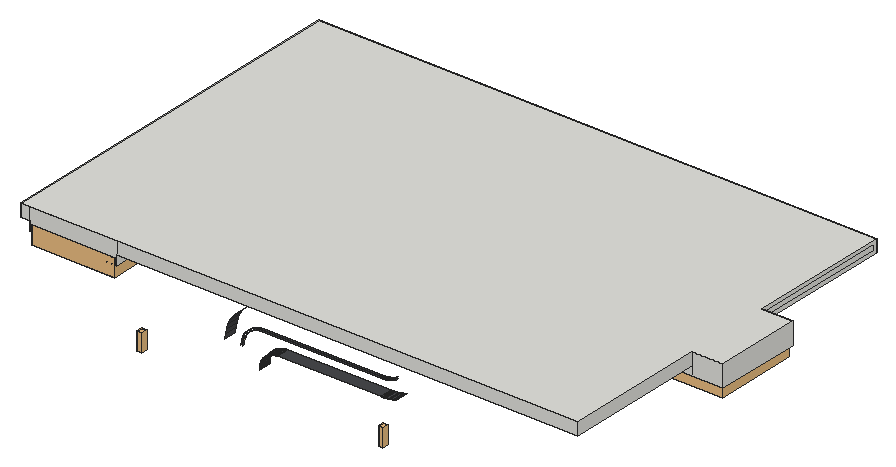
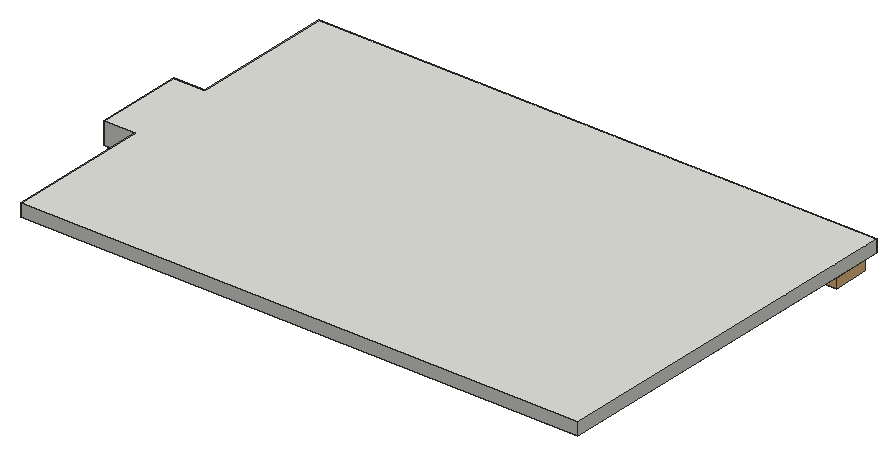
# SketchUp Ruby script. Lengths in inches.
U = 1.inch
M = Sketchup.active_model
def pt(a) = Geom::Point3d.new(a.map { |v| v * U })
def face(e, loops, mat)
  f = e.add_face(loops[0].map { |a| pt(a) })
  loops[1..].each { |l| e.add_face(l.map { |a| pt(a) }).erase! }
  f.material = f.back_material = mat if mat
  f
end
# faces: each face lists its corners as indices into pts; further lists are holes
def faces(e, pts, list, mat = nil) = list.each { |f| face(e, (f[0].is_a?(Array) ? f : [f]).map { |l| l.map { |i| pts[i] } }, mat) }
# xy, xz, yz: faces in a plane at the given z, y or x. An outline is a flat list of corners, or four numbers for a rectangle; further outlines are holes
def ring(l) = l.size == 4 ? [[l[0], l[1]], [l[2], l[1]], [l[2], l[3]], [l[0], l[3]]] : l.each_slice(2).to_a
def flat(e, list, mat, &to3) = list.each { |f| face(e, (f[0].is_a?(Array) ? f : [f]).map { |l| ring(l).map { |u, v| to3.(u, v) } }, mat) }
def xy(e, z, list, mat = nil) = flat(e, list, mat) { |x, y| [x, y, z] }
def xz(e, y, list, mat = nil) = flat(e, list, mat) { |x, z| [x, y, z] }
def yz(e, x, list, mat = nil) = flat(e, list, mat) { |y, z| [x, y, z] }
def lines(e, pts, list) = list.each { |a, b| e.add_line(pt(pts[a]), pt(pts[b])) }
# prism: a flat outline (further loops are holes) pulled along v
def prism(e, loops, v, mat = nil)
  f = face(e, loops, mat); d = Geom::Vector3d.new(v.map { |x| x * U })
  f.pushpull(f.normal.samedirection?(d) ? d.length : -d.length)
end
def box(e, o, s, mat = nil) = prism(e, [[o, [o[0] + s[0], o[1], o[2]], [o[0] + s[0], o[1] + s[1], o[2]], [o[0], o[1] + s[1], o[2]]]], [0, 0, s[2]], mat)
def at(x, y, z, deg = 0) = Geom::Transformation.translation(pt([x, y, z])) * Geom::Transformation.rotation(ORIGIN, Z_AXIS, deg.degrees)
def axes(o, x, y, z) = Geom::Transformation.new([*x, 0, *y, 0, *z, 0, *pt(o).to_a, 1])
def part(name) = M.definitions.add(name)
# library, detail: a bought-in or finely detailed component or shape, given as its bounding box
def library(name, o, s) = part(name).tap { |d| box(d.entities, o, s) }
def detail(e, o, s) = box(e.add_group.entities, o, s)
def put(e, d, t, mat = nil) = e.add_instance(d, t).tap { |i| i.material = mat if mat }
def group(e, t, mat = nil) = e.add_group.tap { |g| g.transformation = t; g.material = mat if mat }.entities
root = M.entities
M.materials.add("1432 AP 8245 TAR ROAD").color = [71, 72, 75]
M.materials.add("Outer Light").color = [251, 217, 152]
c1 = library("WALL LIGHT 69",[4.19,4.05,-8.78],[4.61,5.7,17.13])
c2 = library("Group\#58",[0,0,-17.09],[62,80,17.09])
c3 = library("Group\#32",[0,0,-17.09],[62,80,17.09])
xy(root,266.79,[[282,101.37,284.12,107.37]],"1432 AP 8245 TAR ROAD")
xy(root,269.79,[[293.58,95.37,293.79,107.37],[293.79,95.37,294,107.37],[294,95.37,393,107.37]],"1432 AP 8245 TAR ROAD")
xy(root,285.79,[[279,95.37,393,96.87]],"1432 AP 8245 TAR ROAD")
xy(root,285.79,[[279,95.37,393,96.87]],"Outer Light")
xy(root,285.8,[[393.46,95.37,393.92,96.87]],"1432 AP 8245 TAR ROAD")
xy(root,285.8,[[393.46,95.37,393.92,96.87]],"Outer Light")
xy(root,287.29,[[279,95.37,393,96.87],[393,95.37,393.4375,96.87]],"1432 AP 8245 TAR ROAD")
xy(root,287.29,[[279,95.37,393,96.87],[393,95.37,393.4375,96.87]],"Outer Light")
xz(root,101.37,[[282,265.16,282,266.79,284.12,266.79,283.74,266.55,283.56,266.43,283.37,266.3,283.19,266.17,283.01,266.03,282.84,265.9,282.67,265.76,282.49,265.61,282.33,265.46,282.16,265.3125]],"1432 AP 8245 TAR ROAD")
xz(root,107.37,[[282,265.16,283.04,266.07,284.12,266.79,282,266.79]],"1432 AP 8245 TAR ROAD")
yz(root,276,[[95.37,251.79,107.37,251.99],[95.37,251.99,107.37,252.19]],"1432 AP 8245 TAR ROAD")
yz(root,282,[[101.37,265.16,107.37,266.79]],"1432 AP 8245 TAR ROAD")
p = [[276,107.37,252.19],[276.01,107.37,252.4],[276.01,95.37,252.4],[276,95.37,252.19],[276.02,107.37,252.6],[276.02,95.37,252.6],
  [276.03,107.37,252.8],[276.03,95.37,252.8],[276.04,107.37,253],[276.04,95.37,253],[276.06,107.37,253.2],[276.06,95.37,253.2],
  [276.07,107.37,253.4],[276.07,95.37,253.4],[276.09,107.37,253.6],[276.09,95.37,253.6],[276.11,107.37,253.8],[276.11,95.37,253.8],
  [276.14,107.37,254],[276.14,95.37,254],[276.16,107.37,254.2],[276.16,95.37,254.2],[276.19,107.37,254.4],[276.19,95.37,254.4],
  [276.22,107.37,254.6],[276.22,95.37,254.6],[276.25,107.37,254.8],[276.25,95.37,254.8],[276.29,107.37,255],[276.29,95.37,255],
  [276.32,107.37,255.2],[276.32,95.37,255.2],[276.36,107.37,255.39],[276.36,95.37,255.39],[276.41,107.37,255.59],[276.41,95.37,255.59],
  [276.45,107.37,255.79],[276.45,95.37,255.79],[276.49,107.37,255.98],[276.49,95.37,255.98],[276.54,107.37,256.18],[276.54,95.37,256.18],
  [276.59,107.37,256.375],[276.59,95.37,256.375],[276.65,107.37,256.57],[276.65,95.37,256.57],[276.7,107.37,256.76],[276.7,95.37,256.76],
  [276.76,107.37,256.96],[276.76,95.37,256.96],[276.82,107.37,257.15],[276.82,95.37,257.15],[276.875,107.37,257.34],[276.875,95.37,257.34],
  [276.9375,107.37,257.53],[276.9375,95.37,257.53],[277,107.37,257.72],[277,95.37,257.72],[277.07,107.37,257.91],[277.07,95.37,257.91],
  [277.14,107.37,258.1],[277.14,95.37,258.1],[277.21,107.37,258.29],[277.21,95.37,258.29],[277.29,107.37,258.48],[277.29,95.37,258.48],
  [277.36,107.37,258.66],[277.36,95.37,258.66],[277.44,107.37,258.85],[277.44,95.37,258.85],[277.52,107.37,259.03],[277.52,95.37,259.03],
  [277.6,107.37,259.22],[277.6,95.37,259.22],[277.6875,107.37,259.4],[277.6875,95.37,259.4],[277.77,107.37,259.58],[277.77,95.37,259.58],
  [277.86,107.37,259.76],[277.86,95.37,259.76],[277.95,107.37,259.94],[277.95,95.37,259.94],[278.04,107.37,260.12],[278.04,95.37,260.12],
  [278.14,107.37,260.3],[278.14,95.37,260.3],[278.23,107.37,260.48],[278.23,95.37,260.48],[278.33,107.37,260.65],[278.33,95.37,260.65],
  [278.43,107.37,260.83],[278.43,95.37,260.83],[278.53,107.37,261],[278.53,95.37,261],[278.64,107.37,261.17],[278.64,95.37,261.17],
  [278.74,107.37,261.35],[278.74,95.37,261.35],[278.85,107.37,261.52],[278.85,95.37,261.52],[278.96,107.37,261.68],[278.96,95.37,261.68],
  [279.07,107.37,261.85],[279.07,95.37,261.85],[279.1875,107.37,262.02],[279.1875,95.37,262.02],[279.3,107.37,262.18],[279.3,95.37,262.18],
  [279.42,107.37,262.35],[279.42,95.37,262.35],[279.54,107.37,262.51],[279.54,95.37,262.51],[279.66,107.37,262.67],[279.66,95.37,262.67],
  [279.78,107.37,262.83],[279.78,95.37,262.83],[279.91,107.37,262.99],[279.91,95.37,262.99],[280.03,107.37,263.15],[280.03,95.37,263.15],
  [280.16,107.37,263.3],[280.16,95.37,263.3],[280.29,107.37,263.46],[280.29,95.37,263.46],[280.42,107.37,263.61],[280.42,95.37,263.61],
  [280.55,107.37,263.76],[280.55,95.37,263.76],[280.6875,107.37,263.91],[280.6875,95.37,263.91],[280.83,107.37,264.06],[280.83,95.37,264.06],
  [280.96,107.37,264.2],[280.96,95.37,264.2],[281.1,107.37,264.35],[281.1,95.37,264.35],[281.24,107.37,264.49],[281.24,95.37,264.49],
  [281.39,107.37,264.63],[281.39,95.37,264.63],[281.53,107.37,264.77],[281.53,95.37,264.77],[281.68,107.37,264.91],[281.68,95.37,264.91],
  [281.83,107.37,265.05],[281.83,95.37,265.05],[282,107.37,265.16],[282,101.37,265.16],[282,95.37,265.16],[282.16,95.37,265.3125],
  [282.16,101.37,265.3125],[282.33,95.37,265.46],[282.33,101.37,265.46],[282.49,95.37,265.61],[282.49,101.37,265.61],[282.67,95.37,265.76],
  [282.67,101.37,265.76],[282.84,95.37,265.9],[282.84,101.37,265.9],[283.01,95.37,266.03],[283.01,101.37,266.03],[283.19,95.37,266.17],
  [283.19,101.37,266.17],[283.37,95.37,266.3],[283.37,101.37,266.3],[283.56,95.37,266.43],[283.56,101.37,266.43],[283.74,95.37,266.55],
  [283.74,101.37,266.55],[283.93,95.37,266.67],[283.93,101.37,266.67],[284.12,95.37,266.79],[284.12,101.37,266.79],[243.31,107.37,271.49],
  [243,107.37,266.79],[243,95.37,266.79],[243.31,95.37,271.49],[258.68,95.37,269.47],[258.5,95.37,266.79],[258.5,96.87,266.79],
  [258.68,96.87,269.47],[258.68,96.87,269.47],[258.5,96.87,266.79],[258.5,95.37,266.79],[258.68,95.37,269.47],[260,95.37,266.79],
  [260.16,95.37,269.27],[260.16,96.87,269.27],[260,96.87,266.79],[260,96.87,266.79],[260.16,96.87,269.27],[260.16,95.37,269.27],
  [260,95.37,266.79],[284.12,107.37,266.79],[284.27,107.37,266.9375],[284.27,95.37,266.9375],[284.45,107.37,267.05],[284.45,95.37,267.05],
  [284.63,107.37,267.16],[284.63,95.37,267.16],[284.81,107.37,267.27],[284.81,95.37,267.27],[284.99,107.37,267.375],[284.99,95.37,267.375],
  [285.17,107.37,267.48],[285.17,95.37,267.48],[285.36,107.37,267.58],[285.36,95.37,267.58],[285.54,107.37,267.68],[285.54,95.37,267.68],
  [285.73,107.37,267.78],[285.73,95.37,267.78],[285.91,107.37,267.87],[285.91,95.37,267.87],[286.1,107.37,267.97],[286.1,95.37,267.97],
  [286.29,107.37,268.06],[286.29,95.37,268.06],[286.48,107.37,268.15],[286.48,95.37,268.15],[286.67,107.37,268.23],[286.67,95.37,268.23],
  [286.86,107.37,268.32],[286.86,95.37,268.32],[287.06,107.37,268.4],[287.06,95.37,268.4],[287.25,107.37,268.48],[287.25,95.37,268.48],
  [287.44,107.37,268.56],[287.44,95.37,268.56],[287.64,107.37,268.63],[287.64,95.37,268.63],[287.84,107.37,268.7],[287.84,95.37,268.7],
  [288.03,107.37,268.77],[288.03,95.37,268.77],[288.23,107.37,268.84],[288.23,95.37,268.84],[288.43,107.37,268.91],[288.43,95.37,268.91],
  [288.63,107.37,268.97],[288.63,95.37,268.97],[288.83,107.37,269.03],[288.83,95.37,269.03],[289.03,107.37,269.09],[289.03,95.37,269.09],
  [289.23,107.37,269.15],[289.23,95.37,269.15],[289.4375,107.37,269.2],[289.4375,95.37,269.2],[289.64,107.37,269.26],[289.64,95.37,269.26],
  [260.65,95.37,271.71],[260.65,96.87,271.71],[260.65,96.87,271.71],[260.65,95.37,271.71],[289.84,107.37,269.31],[289.84,95.37,269.31],
  [290.05,107.37,269.35],[290.05,95.37,269.35],[290.25,107.37,269.4],[290.25,95.37,269.4],[290.46,107.37,269.44],[290.46,95.37,269.44],
  [290.66,107.37,269.48],[290.66,95.37,269.48],[259.2,95.37,272.1],[259.2,96.87,272.1],[259.2,96.87,272.1],[259.2,95.37,272.1],
  [290.87,107.37,269.52],[290.87,95.37,269.52],[291.08,107.37,269.55],[291.08,95.37,269.55],[291.28,107.37,269.59],[291.28,95.37,269.59],
  [291.49,107.37,269.62],[291.49,95.37,269.62],[291.7,107.37,269.64],[291.7,95.37,269.64],[291.91,107.37,269.67],[291.91,95.37,269.67],
  [292.12,107.37,269.69],[292.12,95.37,269.69],[292.32,107.37,269.71],[292.32,95.37,269.71],[292.53,107.37,269.73],[292.53,95.37,269.73],
  [292.74,107.37,269.75],[292.74,95.37,269.75],[292.95,107.37,269.76],[292.95,95.37,269.76],[293.16,107.37,269.77],[293.16,95.37,269.77],
  [293.37,107.37,269.78],[293.37,95.37,269.78],[293.58,107.37,269.79],[293.58,95.37,269.79],[393,107.37,269.79],[393.67,107.37,269.8],
  [393.67,95.37,269.8],[393,95.37,269.79],[394.34,107.37,269.81],[394.34,95.37,269.81],[395,107.37,269.83],[395,95.37,269.83],
  [395.67,107.37,269.86],[395.67,95.37,269.86],[396.34,107.37,269.9],[396.34,95.37,269.9],[397,107.37,269.95],[397,95.37,269.95],
  [397.67,107.37,270.01],[397.67,95.37,270.01],[398.33,107.37,270.07],[398.33,95.37,270.07],[398.99,107.37,270.15],[398.99,95.37,270.15],
  [399.66,107.37,270.23],[399.66,95.37,270.23],[400.32,107.37,270.32],[400.32,95.37,270.32],[400.98,107.37,270.42],[400.98,95.37,270.42],
  [401.64,107.37,270.53],[401.64,95.37,270.53],[402.29,107.37,270.65],[402.29,95.37,270.65],[402.95,107.37,270.77],[402.95,95.37,270.77],
  [403.6,107.37,270.91],[403.6,95.37,270.91],[404.26,107.37,271.05],[404.26,95.37,271.05],[404.91,107.37,271.2],[404.91,95.37,271.2],
  [405.55,107.37,271.36],[405.55,95.37,271.36],[406.2,107.37,271.53],[406.2,95.37,271.53],[244.23,107.37,276.11],[244.23,95.37,276.11],
  [406.84,107.37,271.71],[406.84,95.37,271.71],[261.45,95.37,274.0625],[261.45,96.87,274.0625],[261.45,96.87,274.0625],[261.45,95.37,274.0625],
  [407.48,107.37,271.89],[407.48,95.37,271.89],[408.125,107.37,272.09],[408.125,95.37,272.09],[260.06,95.37,274.64],[260.06,96.87,274.64],
  [260.06,96.87,274.64],[260.06,95.37,274.64],[262.55,95.37,276.29],[262.55,96.87,276.29],[262.55,96.87,276.29],[262.55,95.37,276.29],
  [261.25,95.37,277.04],[261.25,96.87,277.04],[261.25,96.87,277.04],[261.25,95.37,277.04],[245.74,107.37,280.57],[245.74,95.37,280.57],
  [263.93,95.37,278.36],[263.93,96.87,278.36],[263.93,96.87,278.36],[263.93,95.37,278.36],[262.74,95.37,279.27],[262.74,96.87,279.27],
  [262.74,96.87,279.27],[262.74,95.37,279.27],[265.56,95.37,280.23],[265.56,96.87,280.23],[265.56,96.87,280.23],[265.56,95.37,280.23],
  [264.5,95.37,281.29],[264.5,96.87,281.29],[264.5,96.87,281.29],[264.5,95.37,281.29],[267.43,95.37,281.87],[267.43,96.87,281.87],
  [267.43,96.87,281.87],[267.43,95.37,281.87],[247.82,107.37,284.79],[247.82,95.37,284.79],[266.52,95.37,283.06],[266.52,96.87,283.06],
  [266.52,96.87,283.06],[266.52,95.37,283.06],[269.5,95.37,283.25],[269.5,96.87,283.25],[269.5,96.87,283.25],[269.5,95.37,283.25],
  [268.75,95.37,284.55],[268.75,96.87,284.55],[268.75,96.87,284.55],[268.75,95.37,284.55],[271.73,95.37,284.35],[271.73,96.87,284.35],
  [271.73,96.87,284.35],[271.73,95.37,284.35],[274.08,95.37,285.14],[274.08,96.87,285.14],[274.08,96.87,285.14],[274.08,95.37,285.14],
  [271.15,95.37,285.73],[271.15,96.87,285.73],[271.15,96.87,285.73],[271.15,95.37,285.73],[250.4375,107.37,288.71],[250.4375,95.37,288.71],
  [276.52,95.37,285.63],[276.52,96.87,285.63],[276.52,96.87,285.63],[276.52,95.37,285.63],[279,95.37,285.79],[279,96.87,285.79],
  [279,96.87,285.79],[279,95.37,285.79],[273.69,95.37,286.59],[273.69,96.87,286.59],[273.69,96.87,286.59],[273.69,95.37,286.59],
  [393,95.37,285.79],[393.46,95.37,285.8],[393.46,96.87,285.8],[393,96.87,285.79],[393,96.87,285.79],[393.46,96.87,285.8],
  [393.46,95.37,285.8],[393,95.37,285.79],[393.92,95.37,285.8],[394.375,95.37,285.82],[394.375,96.87,285.82],[393.92,96.87,285.8],
  [393.92,96.87,285.8],[394.375,96.87,285.82],[394.375,95.37,285.82],[393.92,95.37,285.8],[394.83,95.37,285.84],[394.83,96.87,285.84],
  [394.83,96.87,285.84],[394.83,95.37,285.84],[395.29,95.37,285.87],[395.29,96.87,285.87],[395.29,96.87,285.87],[395.29,95.37,285.87],
  [395.75,95.37,285.9],[395.75,96.87,285.9],[395.75,96.87,285.9],[395.75,95.37,285.9],[396.2,95.37,285.9375],[396.2,96.87,285.9375],
  [396.2,96.87,285.9375],[396.2,95.37,285.9375],[396.66,95.37,285.98],[396.66,96.87,285.98],[396.66,96.87,285.98],[396.66,95.37,285.98],
  [397.11,95.37,286.03],[397.11,96.87,286.03],[397.11,96.87,286.03],[397.11,95.37,286.03],[397.57,95.37,286.09],[397.57,96.87,286.09],
  [397.57,96.87,286.09],[397.57,95.37,286.09],[398.02,95.37,286.15],[398.02,96.87,286.15],[398.02,96.87,286.15],[398.02,95.37,286.15],
  [398.48,95.37,286.22],[398.48,96.87,286.22],[398.48,96.87,286.22],[398.48,95.37,286.22],[398.93,95.37,286.3],[398.93,96.87,286.3],
  [398.93,96.87,286.3],[398.93,95.37,286.3],[399.38,95.37,286.38],[399.38,96.87,286.38],[399.38,96.87,286.38],[399.38,95.37,286.38],
  [399.83,95.37,286.46],[399.83,96.87,286.46],[399.83,96.87,286.46],[399.83,95.37,286.46],[400.28,95.37,286.56],[400.28,96.87,286.56],
  [400.28,96.87,286.56],[400.28,95.37,286.56],[276.32,95.37,287.12],[276.32,96.87,287.12],[276.32,96.87,287.12],[276.32,95.37,287.12],
  [400.72,95.37,286.66],[400.72,96.87,286.66],[400.72,96.87,286.66],[400.72,95.37,286.66],[401.17,95.37,286.76],[401.17,96.87,286.76],
  [401.17,96.87,286.76],[401.17,95.37,286.76],[401.62,95.37,286.87],[401.62,96.87,286.87],[401.62,96.87,286.87],[401.62,95.37,286.87],
  [402.06,95.37,286.98],[402.06,96.87,286.98],[402.06,96.87,286.98],[402.06,95.37,286.98],[402.5,95.37,287.11],[402.5,96.87,287.11],
  [402.5,96.87,287.11],[402.5,95.37,287.11],[279,95.37,287.29],[279,96.87,287.29],[279,96.87,287.29],[279,95.37,287.29],
  [402.94,95.37,287.23],[402.94,96.87,287.23],[402.94,96.87,287.23],[402.94,95.37,287.23],[403.38,95.37,287.37],[403.38,96.87,287.37],
  [403.38,96.87,287.37],[403.38,95.37,287.37],[393.875,95.37,287.3],[393.4375,95.37,287.29],[393.4375,96.87,287.29],[393.875,96.87,287.3],
  [393.875,96.87,287.3],[393.4375,96.87,287.29],[393.4375,95.37,287.29],[393.875,95.37,287.3],[394.32,95.37,287.32],[394.32,96.87,287.32],
  [394.32,96.87,287.32],[394.32,95.37,287.32],[394.75,95.37,287.34],[394.75,96.87,287.34],[394.75,96.87,287.34],[394.75,95.37,287.34],
  [395.19,95.37,287.36],[395.19,96.87,287.36],[395.19,96.87,287.36],[395.19,95.37,287.36],[395.63,95.37,287.4],[395.63,96.87,287.4],
  [395.63,96.87,287.4],[395.63,95.37,287.4],[396.07,95.37,287.43],[396.07,96.87,287.43],[396.07,96.87,287.43],[396.07,95.37,287.43],
  [396.5,95.37,287.48],[396.5,96.87,287.48],[396.5,96.87,287.48],[396.5,95.37,287.48],[403.82,95.37,287.51],[403.82,96.87,287.51],
  [403.82,96.87,287.51],[403.82,95.37,287.51],[396.9375,95.37,287.52],[396.9375,96.87,287.52],[396.9375,96.87,287.52],[396.9375,95.37,287.52],
  [397.37,95.37,287.58],[397.37,96.87,287.58],[397.37,96.87,287.58],[397.37,95.37,287.58],[404.25,95.37,287.65],[404.25,96.87,287.65],
  [404.25,96.87,287.65],[404.25,95.37,287.65],[397.81,95.37,287.64],[397.81,96.87,287.64],[397.81,96.87,287.64],[397.81,95.37,287.64],
  [398.24,95.37,287.7],[398.24,96.87,287.7],[398.24,96.87,287.7],[398.24,95.37,287.7],[404.68,95.37,287.8],[404.68,96.87,287.8],
  [404.68,96.87,287.8],[404.68,95.37,287.8],[398.67,95.37,287.78],[398.67,96.87,287.78],[398.67,96.87,287.78],[398.67,95.37,287.78],
  [399.1,95.37,287.85],[399.1,96.87,287.85],[399.1,96.87,287.85],[399.1,95.37,287.85],[405.11,95.37,287.96],[405.11,96.87,287.96],
  [405.11,96.87,287.96],[405.11,95.37,287.96],[399.54,95.37,287.9375],[399.54,96.87,287.9375],[399.54,96.87,287.9375],[399.54,95.37,287.9375],
  [399.97,95.37,288.02],[399.97,96.87,288.02],[399.97,96.87,288.02],[399.97,95.37,288.02],[400.39,95.37,288.12],[400.39,96.87,288.12],
  [400.39,96.87,288.12],[400.39,95.37,288.12],[405.54,95.37,288.12],[405.54,96.87,288.12],[405.54,96.87,288.12],[405.54,95.37,288.12],
  [400.82,95.37,288.22],[400.82,96.87,288.22],[400.82,96.87,288.22],[400.82,95.37,288.22],[405.97,95.37,288.28],[405.97,96.87,288.28],
  [405.97,96.87,288.28],[405.97,95.37,288.28],[401.25,95.37,288.32],[401.25,96.87,288.32],[401.25,96.87,288.32],[401.25,95.37,288.32],
  [401.67,95.37,288.43],[401.67,96.87,288.43],[401.67,96.87,288.43],[401.67,95.37,288.43],[406.39,95.37,288.46],[406.39,96.87,288.46],
  [406.39,96.87,288.46],[406.39,95.37,288.46],[402.09,95.37,288.55],[402.09,96.87,288.55],[402.09,96.87,288.55],[402.09,95.37,288.55],
  [402.51,95.37,288.67],[402.51,96.87,288.67],[402.51,96.87,288.67],[402.51,95.37,288.67],[406.82,95.37,288.63],[406.82,96.87,288.63],
  [406.82,96.87,288.63],[406.82,95.37,288.63],[407.24,95.37,288.82],[407.24,96.87,288.82],[407.24,96.87,288.82],[407.24,95.37,288.82],
  [253.54,107.37,292.25],[253.54,95.37,292.25],[402.93,95.37,288.8],[402.93,96.87,288.8],[402.93,96.87,288.8],[402.93,95.37,288.8],
  [403.35,95.37,288.93],[403.35,96.87,288.93],[403.35,96.87,288.93],[403.35,95.37,288.93],[407.65,95.37,289.01],[407.65,96.87,289.01],
  [407.65,96.87,289.01],[407.65,95.37,289.01],[403.77,95.37,289.07],[403.77,96.87,289.07],[403.77,96.87,289.07],[403.77,95.37,289.07],
  [408.07,95.37,289.2],[408.07,96.87,289.2],[408.07,96.87,289.2],[408.07,95.37,289.2],[404.18,95.37,289.21],[404.18,96.87,289.21],
  [404.18,96.87,289.21],[404.18,95.37,289.21],[404.59,95.37,289.36],[404.59,96.87,289.36],[404.59,96.87,289.36],[404.59,95.37,289.36],
  [405.01,95.37,289.52],[405.01,96.87,289.52],[405.01,96.87,289.52],[405.01,95.37,289.52],[405.41,95.37,289.68],[405.41,96.87,289.68],
  [405.41,96.87,289.68],[405.41,95.37,289.68],[405.82,95.37,289.84],[405.82,96.87,289.84],[405.82,96.87,289.84],[405.82,95.37,289.84],
  [406.22,95.37,290.01],[406.22,96.87,290.01],[406.22,96.87,290.01],[406.22,95.37,290.01],[406.625,95.37,290.1875],[406.625,96.87,290.1875],
  [406.625,96.87,290.1875],[406.625,95.37,290.1875],[407.03,95.37,290.37],[407.03,96.87,290.37],[407.03,96.87,290.37],[407.03,95.37,290.37],
  [407.42,95.37,290.56],[407.42,96.87,290.56],[407.42,96.87,290.56],[407.42,95.37,290.56],[407.82,95.37,290.75],[407.82,96.87,290.75],
  [407.82,96.87,290.75],[407.82,95.37,290.75],[408.21,95.37,290.94],[408.21,96.87,290.94],[257.08,107.37,295.35],[257.08,95.37,295.35],
  [282,101.37,266.79],[282,95.37,266.79]]
faces(root,p,[[0,1,2,3],[1,4,5,2],[4,6,7,5],[6,8,9,7],[8,10,11,9],[10,12,13,11],[12,14,15,13],[14,16,17,15],
  [16,18,19,17],[18,20,21,19],[20,22,23,21],[22,24,25,23],[24,26,27,25],[26,28,29,27],[28,30,31,29],[30,32,33,31],
  [32,34,35,33],[34,36,37,35],[36,38,39,37],[38,40,41,39],[40,42,43,41],[42,44,45,43],[44,46,47,45],[46,48,49,47],
  [48,50,51,49],[50,52,53,51],[52,54,55,53],[54,56,57,55],[56,58,59,57],[58,60,61,59],[60,62,63,61],[62,64,65,63],
  [64,66,67,65],[66,68,69,67],[68,70,71,69],[70,72,73,71],[72,74,75,73],[74,76,77,75],[76,78,79,77],[78,80,81,79],
  [80,82,83,81],[82,84,85,83],[84,86,87,85],[86,88,89,87],[88,90,91,89],[90,92,93,91],[92,94,95,93],[94,96,97,95],
  [96,98,99,97],[98,100,101,99],[100,102,103,101],[102,104,105,103],[104,106,107,105],[106,108,109,107],[108,110,111,109],[110,112,113,111],
  [112,114,115,113],[114,116,117,115],[116,118,119,117],[118,120,121,119],[120,122,123,121],[122,124,125,123],[124,126,127,125],[126,128,129,127],
  [128,130,131,129],[130,132,133,131],[132,134,135,133],[134,136,137,135],[136,138,139,137],[138,140,141,139],[140,142,143,141],[142,144,145,143],
  [144,146,147,148,145],[149,148,147,150],[151,149,150,152],[153,151,152,154],[155,153,154,156],[157,155,156,158],[159,157,158,160],[161,159,160,162],
  [163,161,162,164],[165,163,164,166],[167,165,166,168],[169,167,168,170],[171,169,170,172],[173,174,175,176],[177,178,179,180],[185,186,187,188],
  [193,194,195,171,172],[194,196,197,195],[196,198,199,197],[198,200,201,199],[200,202,203,201],[202,204,205,203],[204,206,207,205],[206,208,209,207],
  [208,210,211,209],[210,212,213,211],[212,214,215,213],[214,216,217,215],[216,218,219,217],[218,220,221,219],[220,222,223,221],[222,224,225,223],
  [224,226,227,225],[226,228,229,227],[228,230,231,229],[230,232,233,231],[232,234,235,233],[234,236,237,235],[236,238,239,237],[238,240,241,239],
  [240,242,243,241],[242,244,245,243],[244,246,247,245],[246,248,249,247],[248,250,251,249],[186,252,253,187],[250,256,257,251],[256,258,259,257],
  [258,260,261,259],[260,262,263,261],[262,264,265,263],[266,177,180,267],[264,270,271,265],[270,272,273,271],[272,274,275,273],[274,276,277,275],
  [276,278,279,277],[278,280,281,279],[280,282,283,281],[282,284,285,283],[284,286,287,285],[286,288,289,287],[288,290,291,289],[290,292,293,291],
  [292,294,295,293],[294,296,297,295],[298,299,300,301],[299,302,303,300],[302,304,305,303],[304,306,307,305],[306,308,309,307],[308,310,311,309],
  [310,312,313,311],[312,314,315,313],[314,316,317,315],[316,318,319,317],[318,320,321,319],[320,322,323,321],[322,324,325,323],[324,326,327,325],
  [326,328,329,327],[328,330,331,329],[330,332,333,331],[332,334,335,333],[334,336,337,335],[336,338,339,337],[340,173,176,341],[338,342,343,339],
  [252,344,345,253],[342,348,349,343],[348,350,351,349],[352,266,267,353],[344,356,357,345],[360,352,353,361],[364,340,341,365],[356,366,367,357],
  [370,360,361,371],[366,374,375,367],[378,370,371,379],[374,382,383,375],[386,364,365,387],[388,378,379,389],[382,392,393,383],[396,388,389,397],
  [392,400,401,393],[400,404,405,401],[408,396,397,409],[412,386,387,413],[404,414,415,405],[414,418,419,415],[422,408,409,423],[426,427,428,429],
  [434,435,436,437],[435,442,443,436],[442,446,447,443],[446,450,451,447],[450,454,455,451],[454,458,459,455],[458,462,463,459],[462,466,467,463],
  [466,470,471,467],[470,474,475,471],[474,478,479,475],[478,482,483,479],[482,486,487,483],[486,490,491,487],[494,422,423,495],[490,498,499,491],
  [498,502,503,499],[502,506,507,503],[506,510,511,507],[510,514,515,511],[518,494,495,519],[514,522,523,515],[522,526,527,523],[530,531,532,533],
  [538,530,533,539],[542,538,539,543],[546,542,543,547],[550,546,547,551],[554,550,551,555],[558,554,555,559],[526,562,563,527],[566,558,559,567],
  [570,566,567,571],[562,574,575,563],[578,570,571,579],[582,578,579,583],[574,586,587,575],[590,582,583,591],[594,590,591,595],[586,598,599,587],
  [602,594,595,603],[606,602,603,607],[610,606,607,611],[598,614,615,599],[618,610,611,619],[614,622,623,615],[626,618,619,627],[630,626,627,631],
  [622,634,635,623],[638,630,631,639],[642,638,639,643],[634,646,647,635],[646,650,651,647],[654,412,413,655],[656,642,643,657],[660,656,657,661],
  [650,664,665,651],[668,660,661,669],[664,672,673,665],[676,668,669,677],[680,676,677,681],[684,680,681,685],[688,684,685,689],[692,688,689,693],
  [696,692,693,697],[700,696,697,701],[704,700,701,705],[708,704,705,709],[712,708,709,713],[716,712,713,717],[718,654,655,719]],"1432 AP 8245 TAR ROAD")
faces(root,p,[[181,182,183,184],[189,190,191,192],[190,254,255,191],[268,181,184,269],[254,346,347,255],[354,268,269,355],[346,358,359,347],[362,354,355,363],
  [358,368,369,359],[372,362,363,373],[368,376,377,369],[380,372,373,381],[376,384,385,377],[390,380,381,391],[384,394,395,385],[398,390,391,399],
  [394,402,403,395],[402,406,407,403],[410,398,399,411],[406,416,417,407],[416,420,421,417],[424,410,411,425],[430,431,432,433],[438,439,440,441],
  [439,444,445,440],[444,448,449,445],[448,452,453,449],[452,456,457,453],[456,460,461,457],[460,464,465,461],[464,468,469,465],[468,472,473,469],
  [472,476,477,473],[476,480,481,477],[480,484,485,481],[484,488,489,485],[488,492,493,489],[496,424,425,497],[492,500,501,493],[500,504,505,501],
  [504,508,509,505],[508,512,513,509],[512,516,517,513],[520,496,497,521],[516,524,525,517],[524,528,529,525],[534,535,536,537],[540,534,537,541],
  [544,540,541,545],[548,544,545,549],[552,548,549,553],[556,552,553,557],[560,556,557,561],[528,564,565,529],[568,560,561,569],[572,568,569,573],
  [564,576,577,565],[580,572,573,581],[584,580,581,585],[576,588,589,577],[592,584,585,593],[596,592,593,597],[588,600,601,589],[604,596,597,605],
  [608,604,605,609],[612,608,609,613],[600,616,617,601],[620,612,613,621],[616,624,625,617],[628,620,621,629],[632,628,629,633],[624,636,637,625],
  [640,632,633,641],[644,640,641,645],[636,648,649,637],[648,652,653,649],[658,644,645,659],[662,658,659,663],[652,666,667,653],[670,662,663,671],
  [666,674,675,667],[678,670,671,679],[682,678,679,683],[686,682,683,687],[690,686,687,691],[694,690,691,695],[698,694,695,699],[702,698,699,703],
  [706,702,703,707],[710,706,707,711],[714,710,711,715]],"Outer Light")
lines(root,p,[[720,721]])
put(root,c1,at(148.76,97.62,230.66))
g1 = group(root,at(45,116.37,293.79))
xy(g1,-9,[[[0,-9,84,27],[2,-7,82,25]],[[492,129,558,213],[494,131,556,211]]])
xy(g1,-3,[[2,-7,82,25]])
xy(g1,-2,[[494,131,556,211]])
xy(g1,0,[[-9,-9,-9,351,528,351,528,213,492,213,492,129,528,129,528,-9,84,-9,84,27,0,27,0,-9]])
xy(g1,12,[[-9,-9,528,-9,528,129,558,129,558,213,528,213,528,351,-9,351]])
xz(g1,-9,[[0,-9,84,12],[-9,0,0,12],[84,0,528,12]])
xz(g1,-7,[[2,-9,82,-3]])
xz(g1,25,[[2,-9,82,-3]])
xz(g1,27,[[0,-9,84,0]])
xz(g1,129,[[492,-9,528,0],[528,-9,558,12]])
xz(g1,131,[[494,-9,556,-2]])
xz(g1,211,[[494,-9,556,-2]])
xz(g1,213,[[492,-9,528,0],[528,-9,558,12]])
xz(g1,351,[[-9,0,528,12]])
yz(g1,-9,[[-9,0,351,12]])
yz(g1,0,[[-9,-9,27,0]])
yz(g1,2,[[-7,-9,25,-3]])
yz(g1,82,[[-7,-9,25,-3]])
yz(g1,84,[[-9,-9,27,0]])
yz(g1,492,[[129,-9,213,0]])
yz(g1,494,[[131,-9,211,-2]])
yz(g1,528,[[-9,0,129,12],[[213,0,351,12],[216.39,3.39,347.61,8.61]],[216.39,3.39,347.61,8.61]])
yz(g1,556,[[131,-9,211,-2]])
yz(g1,558,[[129,-9,213,12]])
put(g1,c2,at(494,131,-2))
put(g1,c3,axes([2,25,-3],[0,-0.54839,0],[1,0,0],[0,0,1]))
put(root,c1,at(381.51,97.62,230.66))
